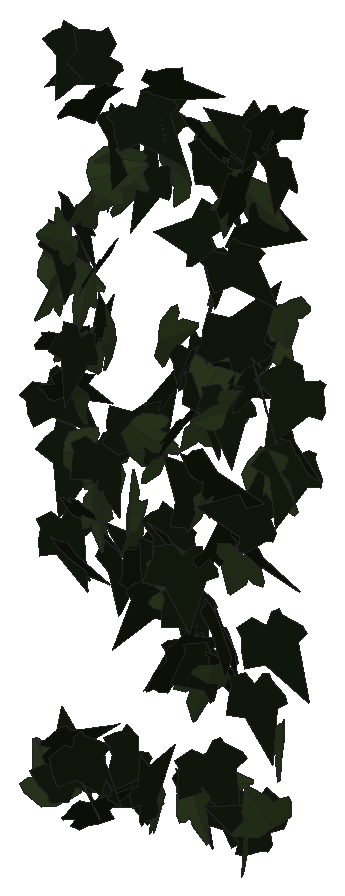
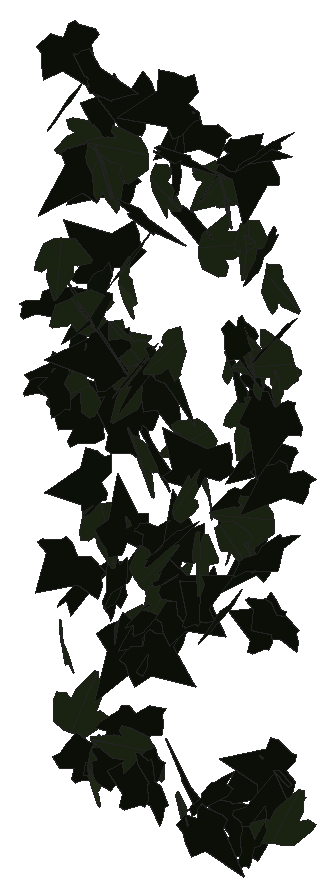
# SketchUp Ruby script. Lengths in inches.
U = 1.inch
M = Sketchup.active_model
def pt(a) = Geom::Point3d.new(a.map { |v| v * U })
def face(e, loops, mat)
  f = e.add_face(loops[0].map { |a| pt(a) })
  loops[1..].each { |l| e.add_face(l.map { |a| pt(a) }).erase! }
  f.material = f.back_material = mat if mat
  f
end
# faces: each face lists its corners as indices into pts; further lists are holes
def faces(e, pts, list, mat = nil) = list.each { |f| face(e, (f[0].is_a?(Array) ? f : [f]).map { |l| l.map { |i| pts[i] } }, mat) }
# xy, xz, yz: faces in a plane at the given z, y or x. An outline is a flat list of corners, or four numbers for a rectangle; further outlines are holes
def ring(l) = l.size == 4 ? [[l[0], l[1]], [l[2], l[1]], [l[2], l[3]], [l[0], l[3]]] : l.each_slice(2).to_a
def flat(e, list, mat, &to3) = list.each { |f| face(e, (f[0].is_a?(Array) ? f : [f]).map { |l| ring(l).map { |u, v| to3.(u, v) } }, mat) }
def xy(e, z, list, mat = nil) = flat(e, list, mat) { |x, y| [x, y, z] }
def xz(e, y, list, mat = nil) = flat(e, list, mat) { |x, z| [x, y, z] }
def yz(e, x, list, mat = nil) = flat(e, list, mat) { |y, z| [x, y, z] }
def lines(e, pts, list) = list.each { |a, b| e.add_line(pt(pts[a]), pt(pts[b])) }
# prism: a flat outline (further loops are holes) pulled along v
def prism(e, loops, v, mat = nil)
  f = face(e, loops, mat); d = Geom::Vector3d.new(v.map { |x| x * U })
  f.pushpull(f.normal.samedirection?(d) ? d.length : -d.length)
end
def box(e, o, s, mat = nil) = prism(e, [[o, [o[0] + s[0], o[1], o[2]], [o[0] + s[0], o[1] + s[1], o[2]], [o[0], o[1] + s[1], o[2]]]], [0, 0, s[2]], mat)
def at(x, y, z, deg = 0) = Geom::Transformation.translation(pt([x, y, z])) * Geom::Transformation.rotation(ORIGIN, Z_AXIS, deg.degrees)
def axes(o, x, y, z) = Geom::Transformation.new([*x, 0, *y, 0, *z, 0, *pt(o).to_a, 1])
def part(name) = M.definitions.add(name)
# library, detail: a bought-in or finely detailed component or shape, given as its bounding box
def library(name, o, s) = part(name).tap { |d| box(d.entities, o, s) }
def detail(e, o, s) = box(e.add_group.entities, o, s)
def put(e, d, t, mat = nil) = e.add_instance(d, t).tap { |i| i.material = mat if mat }
def group(e, t, mat = nil) = e.add_group.tap { |g| g.transformation = t; g.material = mat if mat }.entities
root = M.entities
M.materials.add("efeu1").color = [18, 25, 13]
M.materials.add("efeu2").color = [43, 57, 29]
c1 = part("ivyleaf_9")
p = [[1.54,2.16,1.25],[1.36,2.04,1.19],[-0.21,0.99,0.68],[-0.71,1.11,0.82],[-0.85,0.86,0.67],[-0.8,0.17,0.21],
  [-0.9,-0.01,0.1],[-0.67,-0.16,-0.02],[-0.08,-0.08,-0.05],[-0.03,-0.6,-0.4],[0.65,-0.88,-0.66],[0.83,-0.6,-0.49],
  [1.29,-0.42,-0.43],[1.8125,-0.07,-0.26],[1.21,0.44,0.15]]
faces(c1.entities,p,[[0,1,2,3,4,5,6,7,8,9,10,11,12,13,14]],"efeu1")
c2 = part("ivyleaf_10")
p = [[0,0.5,-0.03],[-0.0625,2.02,-0.43],[-0.19,2.01,-0.46],[-0.54,1.05,-0.29],[-0.52,0.625,-0.18],[-0.83,0.76,-0.28],
  [-1.16,0.64,-0.33],[-1.15,0.33,-0.24],[-0.77,-0.39,0.02],[-0.3,-0.51,0.16],[0.04,-0.48,0.23],[-0.02,2.01,-0.4375],
  [-0.06,2.01,-0.43],[0.04,-0.49,0.23],[0.67,-0.49,0.14],[1.38,0.36,-0.2],[1.375,0.51,-0.24],[0.81,0.65,-0.19],
  [0.62,0.59,-0.15],[0.6,1.09,-0.28],[0.5,1.23,-0.31]]
faces(c2.entities,p,[[0,1,2,3,4,5,6,7,8,9,10],[11,12,0,13,14,15,16,17,18,19,20]],"efeu2")
put(root,c1,axes([566.55,125.93,235.69],[0.48695,-0.82806,0.32776],[0.14634,-0.29408,-0.96038],[0.87846,0.508,-0.0217]))
put(root,c1,axes([576.53,125.82,215.84],[0.2139,-1.10488,-0.24681],[-0.04324,0.24302,-1.12539],[1.13129,0.2182,0.00365]))
put(root,c2,axes([566.59,125.89,226.53],[-0.60718,0.06455,0.81247],[0.77355,-0.27349,0.59981],[0.25672,0.97672,0.11426]))
put(root,c2,axes([570.2,125.27,222.05],[0.76688,-0.41695,0.66634],[-0.54996,0.38051,0.87104],[-0.56161,-0.94198,0.05691]))
put(root,c2,axes([569.02,125.73,238.55],[0.64031,-0.81411,-0.13122],[-0.06589,0.11509,-1.03557],[0.82198,0.6434,0.01921]))
put(root,c2,axes([566.38,125.54,234.33],[-0.24169,0.05211,0.98861],[-0.9899,0.00032,-0.24202],[-0.01269,-1.01773,0.05054]))
put(root,c1,axes([575.42,125.39,236.79],[-0.1494,-0.23257,-1.00547],[0.54358,0.84586,-0.27642],[0.87725,-0.56374,0.00004]))
put(root,c2,axes([568.43,125.38,238.32],[0.39007,-0.07838,-0.94898],[0.92972,0.25294,0.36126],[0.20575,-0.99435,0.1667]))
put(root,c2,axes([568.24,126.27,229.74],[-0.30866,0.37768,0.92115],[0.60809,-0.69208,0.48752],[0.78828,0.68177,-0.0154]))
put(root,c1,axes([573.6,126.06,224.64],[0.40899,-0.33145,1.27453],[1.0095,-0.77814,-0.52631],[0.84571,1.08914,0.01185]))
put(root,c1,axes([576.58,126.56,223.89],[-0.20394,-0.14405,1.19482],[-0.97775,-0.68673,-0.24968],[0.70168,-0.99879,-0.00065]))
put(root,c1,axes([566.02,125.15,209.54],[0.25416,0.7736,-0.6093],[0.12603,0.59854,0.81251],[0.97664,-0.27856,0.05372]))
put(root,c1,axes([566.63,126.13,229.29],[-0.79593,-0.23059,-0.56353],[0.55679,0.09972,-0.82721],[0.24642,-0.97012,0.04892]))
put(root,c1,axes([566.72,125.64,209.44],[-0.18209,-0.27365,-1.02257],[0.61599,0.81643,-0.32817],[0.86087,-0.64207,0.01853]))
put(root,c2,axes([567.29,126.3,221.61],[0.71805,-0.30645,0.80688],[0.75671,-0.28134,-0.78025],[0.41516,1.04283,0.02661]))
put(root,c2,axes([574.77,126.66,228.54],[0.04325,0.06862,-1.05561],[-0.6146,-0.85825,-0.08097],[-0.86097,0.61611,0.00477]))
put(root,c2,axes([567.42,125.78,236.6],[-0.02899,-0.93369,-0.40921],[0.04456,0.40782,-0.93368],[1.01845,-0.04442,0.0292]))
put(root,c1,axes([575.56,125.26,239.25],[0.0199,-0.13283,1.13701],[0.46635,1.03948,0.11327],[-1.04545,0.46116,0.07217]))
put(root,c1,axes([567.06,125.57,206.29],[0.42568,0.88116,-0.3023],[0.13152,0.27219,0.97859],[0.92224,-0.44554,-0.00002]))
put(root,c1,axes([575.42,125.49,232.03],[-0.39089,-0.25075,1.19291],[1.07257,0.52453,0.46171],[-0.57923,1.14048,0.04993]))
put(root,c2,axes([565.49,126.1,206.94],[0.54037,1.0486,0.35028],[-0.1768,-0.3029,1.17951],[1.09133,-0.56828,0.01765]))
put(root,c2,axes([576.62,126.57,209.03],[-0.61666,-0.76684,-0.5738],[-0.36437,-0.44329,0.98402],[-0.88573,0.71625,-0.00531]))
put(root,c1,axes([572.86,127.04,215.16],[-0.33751,-0.47663,1.00169],[-0.09803,-1.03012,-0.52318],[1.10497,-0.23698,0.25955]))
put(root,c1,axes([572.33,126.0625,227.39],[-0.40754,0.83497,-0.34004],[0.1324,-0.31369,-0.92895],[-0.89178,-0.42815,0.01748]))
put(root,c2,axes([568.79,125.87,238.98],[-0.73084,-0.35841,-0.61342],[0.55355,0.26436,-0.81398],[0.44533,-0.9168,0.00509]))
put(root,c1,axes([568.41,127.04,239.49],[0.02553,-0.91032,0.80064],[0.06943,-0.79841,-0.90999],[1.21033,0.065,0.03531]))
put(root,c1,axes([572.02,126.47,220.29],[-0.37583,-0.89923,-0.48626],[0.23868,0.42658,-0.97333],[0.99403,-0.44241,0.04986]))
put(root,c1,axes([566.43,126.08,207.5],[-0.81879,-0.63423,0.4677],[0.36984,0.28629,1.03569],[-0.69585,0.89844,0.00014]))
put(root,c1,axes([574.4,126.52,228.99],[-0.60036,-0.48133,-0.70867],[0.63785,0.32653,-0.76214],[0.57187,-0.8695,0.10609]))
put(root,c2,axes([573.34,126.6,215.01],[-0.27552,-1.10426,0.25761],[-0.0469,-0.25378,-1.13801],[1.13294,-0.27905,0.01554]))
put(root,c1,axes([566.44,126.06,221.1],[1.0125,-0.01233,-0.06006],[-0.05991,0.01285,-1.0125],[0.01307,1.0142,0.0121]))
put(root,c2,axes([567.98,125.74,221.92],[-0.41154,0.56329,0.78885],[-0.44282,0.6531,-0.69737],[-0.86226,-0.60426,-0.01837]))
put(root,c2,axes([572.39,126.54,208.76],[0.75051,-0.12421,0.72321],[0.72656,-0.01921,-0.75729],[0.10285,1.04209,0.07224]))
put(root,c1,axes([573.55,127.12,217.18],[0.22616,-0.7876,0.74488],[0.22085,-0.71148,-0.81935],[1.06131,0.31588,0.01177]))
put(root,c1,axes([572.89,125.99,223.88],[-0.66822,0.17931,-0.96748],[-0.97464,0.03991,0.68057],[0.13507,1.17513,0.12451]))
put(root,c1,axes([573.9,127.12,216.33],[-0.02798,-0.17929,1.15073],[0.38083,-1.08919,-0.16044],[1.10058,0.37233,0.08478]))
put(root,c2,axes([564.68,127.11,230.85],[-0.12079,0.38531,-0.91012],[-0.08997,-0.91737,-0.37644],[-0.98422,0.03657,0.14611]))
put(root,c1,axes([572.1,125.44,215.76],[-0.21963,0.51256,-1.13394],[-0.48694,1.02425,0.5573],[1.14518,0.53383,0.01949]))
put(root,c1,axes([567.19,126.67,223.98],[0.16706,-0.9687,-0.45375],[-0.04865,0.4519,-0.98265],[1.0686,0.17201,0.0262]))
put(root,c1,axes([572.7,126.8,241.17],[0.54792,-0.47737,0.79131],[0.68274,-0.41089,-0.72063],[0.62282,0.87038,0.09381]))
put(root,c1,axes([576.93,126.91,243.52],[-0.03947,0.6301,-0.86428],[0.08915,-0.85992,-0.631],[-1.06586,-0.09526,-0.02077]))
put(root,c1,axes([569.62,126.46,241.48],[-0.05261,-0.49736,-0.98113],[0.53907,0.84456,-0.45703],[0.95885,-0.5021,0.20311]))
put(root,c2,axes([572.93,126.75,224.26],[1.03754,-0.62532,-0.1728],[-0.1373,0.10691,-1.21124],[0.63406,1.04639,0.02048]))
put(root,c2,axes([566.25,126.95,231.75],[1.07502,-0.563,0.17863],[0.16841,-0.06341,-1.21333],[0.56615,1.08792,0.02172]))
put(root,c1,axes([565.42,126.14,226.72],[0.79539,0.4763,0.35874],[0.31504,0.1721,-0.927],[-0.50627,0.85541,-0.01324]))
put(root,c2,axes([569.68,126.48,225.85],[-0.52176,-0.24041,-0.78625],[0.74838,0.24674,-0.57207],[0.34047,-0.91079,0.05256]))
put(root,c1,axes([575.82,126.51,241.78],[-0.35768,0.23247,1.0327],[-0.81807,0.63106,-0.4254],[-0.67177,-0.89228,-0.03181]))
put(root,c2,axes([576.09,126.71,226.08],[0.68938,0.09709,0.99761],[0.96687,0.25479,-0.69293],[-0.26425,1.18556,0.06722]))
put(root,c1,axes([565.89,127.39,206.74],[0.28335,-0.56852,0.83965],[0.35633,-0.76039,-0.6351],[0.94934,0.45509,-0.01223]))
put(root,c2,axes([576.76,127.2,213.05],[0.61421,-0.43975,0.62161],[0.52256,-0.33742,-0.75505],[0.55381,0.8061,0.02305]))
put(root,c1,axes([569.95,127.41,217.7],[-0.0935,0.32339,-1.06895],[0.29821,-1.02651,-0.33663],[-1.07624,-0.31252,-0.00041]))
put(root,c1,axes([572.625,127.24,228.53],[0.34899,-1.02825,0.09986],[0.01563,-0.10014,-1.08573],[1.03297,0.34891,-0.01731]))
put(root,c2,axes([573.16,126.42,227.4],[-0.44802,-0.72054,-0.65323],[0.34786,0.55291,-0.84846],[0.90823,-0.56721,0.00274]))
put(root,c1,axes([575.7,127.59,228.48],[-0.0528,-0.18333,1.15102],[0.27958,-1.12055,-0.16565],[1.1315,0.26833,0.09464]))
put(root,c1,axes([571.6875,126.7,229.11],[-0.73745,0.85299,0.01221],[-0.01628,0.00207,-1.12752],[-0.85292,-0.73755,0.01097]))
put(root,c1,axes([577.68,127.57,230.38],[-0.65017,-0.90154,0.15842],[-0.08946,-0.13081,-1.11152],[0.91097,-0.65628,0.00392]))
put(root,c1,axes([565.24,127.1,217.77],[0.47213,-0.42368,0.70592],[0.59946,-0.38089,-0.62953],[0.56434,0.75905,0.07813]))
put(root,c1,axes([575.04,126.9,221.74],[0.88268,-0.36713,0.45083],[0.42271,-0.15749,-0.95586],[0.39919,0.97856,0.01531]))
put(root,c1,axes([572.99,127.14,240.24],[0.63784,-1.0423,-0.19078],[-0.10369,0.16021,-1.22197],[1.05453,0.6462,-0.00477]))
put(root,c1,axes([569.46,126.87,207.31],[-0.4334,0.76744,0.77397],[0.38828,-0.66955,0.88133],[1.01844,0.58185,-0.00665]))
put(root,c2,axes([567.88,127.86,236.55],[-0.00058,-0.21122,1.13229],[-0.06324,-1.13057,-0.21093],[1.15008,-0.06228,-0.01103]))
put(root,c1,axes([577.27,127.5625,226.59],[-0.43705,-0.97645,-0.02745],[0.01193,0.02474,-1.0698],[0.97676,-0.43721,0.00078]))
put(root,c1,axes([569.82,127.57,220.05],[1.08973,-0.28345,-0.41835],[0.40627,-0.09994,1.12597],[-0.3005,-1.16298,0.0052]))
put(root,c2,axes([575.33,127.05,239.0625],[-0.59983,0.10924,-0.86829],[0.85577,-0.14699,-0.60967],[-0.18307,-1.04504,-0.00501]))
put(root,c1,axes([566.54,126.59,240.9],[0.26965,0.98217,-0.04078],[-0.01633,-0.03781,-1.0185],[-0.98288,0.27008,0.00573]))
put(root,c1,axes([572.92,127.07,236.15],[-0.69091,0.40119,0.58922],[-0.57644,0.16828,-0.79051],[-0.41935,-0.89232,0.11584]))
put(root,c1,axes([572.99,126.93,210.64],[-0.03243,-0.78656,-0.84268],[0.02364,0.84238,-0.78719],[1.15249,-0.03941,-0.00757]))
put(root,c1,axes([564.71,127.7,232.78],[0.06963,-0.96869,0.27036],[0.04177,-0.26799,-0.97094],[1.00484,0.07826,0.02162]))
put(root,c1,axes([576.2,127.82,240.77],[0.12115,-0.89375,0.53404],[0.07342,-0.52897,-0.90193],[1.03856,0.14165,0.00146]))
put(root,c1,axes([565.33,126.7,228.8],[0.63514,0.83868,-0.24486],[-0.16379,-0.18307,-1.05185],[-0.8582,0.65562,0.01953]))
put(root,c2,axes([565.97,127.02,230.13],[0.68303,-0.65518,0.33657],[-0.25092,0.22459,0.9464],[-0.69252,-0.72758,-0.01094]))
put(root,c1,axes([570.49,128.01,220.54],[-0.26353,-0.92701,0.44825],[-0.07262,-0.44481,-0.9626],[1.02713,-0.26929,0.04695]))
put(root,c2,axes([565.83,126.99,223.17],[-0.05377,-0.07689,-1.07137],[1.0559,0.193,-0.06684],[0.19705,-1.05522,0.06584]))
put(root,c2,axes([572.98,126.95,228.9375],[0.87522,0.18903,-0.49509],[0.45765,0.21239,0.89012],[0.26722,-0.98286,0.09713]))
put(root,c1,axes([564.36,126.95,225.89],[0.02578,-0.44563,-0.93884],[0.24069,0.91615,-0.42826],[1.01098,-0.20675,0.1259]))
put(root,c1,axes([567.33,126.5625,229.5625],[-0.07228,0.46618,0.92228],[-0.22421,0.89543,-0.47018],[-1.00879,-0.23242,0.03842]))
put(root,c2,axes([574.53,127.96,207.79],[0.47362,-0.64672,0.95066],[0.667,-0.68294,-0.79689],[0.93654,0.81343,0.08678]))
put(root,c1,axes([565.16,128.0625,242.35],[-0.33346,-0.89236,0.41066],[0.04507,-0.44712,-0.93499],[0.98128,-0.28271,0.1825]))
put(root,c1,axes([575.55,127.82,207.61],[-0.11922,0.01372,1.05028],[-0.98065,-0.38015,-0.10635],[0.37631,-0.9863,0.05559]))
put(root,c1,axes([574.34,127.7,208.23],[-0.24472,-0.24105,-0.9004],[-0.53737,-0.72416,0.33992],[-0.76161,0.5884,0.04948]))
put(root,c1,axes([569.67,127.89,240.3],[0.2498,-0.14624,-1.14518],[1.11616,-0.2688,0.2778],[-0.295,-1.14087,0.08134]))
put(root,c1,axes([567.43,128.03,217.83],[0.0807,-0.88599,0.51674],[0.13376,-0.50481,-0.88645],[1.01691,0.13671,0.07559]))
put(root,c1,axes([568.14,128.1,208.74],[-0.28832,-0.7516,0.52577],[-0.20018,-0.48629,-0.80494],[0.89514,-0.35084,-0.01066]))
put(root,c2,axes([570.04,127.35,207.32],[0.5771,-0.74826,-0.2803],[-0.16599,0.22596,-0.94494],[0.78161,0.60046,0.00629]))
put(root,c2,axes([566.09,127.18,228.65],[-0.60754,-0.84557,-0.34477],[0.1746,0.2989,-1.04074],[0.89631,-0.63137,-0.03096]))
put(root,c1,axes([575.96,127.39,217.84],[-0.32485,-0.39276,-1.11955],[0.85668,0.7254,-0.50306],[0.82082,-0.91253,0.08196]))
put(root,c1,axes([570.15,126.9,242.66],[0.74265,0.21526,0.69483],[0.66982,0.18485,-0.77319],[-0.28366,1.00007,-0.00665]))
put(root,c1,axes([564.54,127.5625,218.97],[-0.35539,-0.36584,-0.94495],[0.84571,0.4445,-0.49016],[0.55816,-0.90645,0.14102]))
put(root,c1,axes([575.66,127,230.43],[-0.81261,0.88012,0.56704],[-0.3647,0.43489,-1.19764],[-0.9814,-0.89036,-0.02446]))
put(root,c2,axes([569.03,127.14,220.78],[0.14913,-0.9081,-0.59435],[-0.13956,0.57891,-0.91952],[1.0763,0.20089,-0.03688]))
put(root,c2,axes([573.96,127.77,238.4],[0.0177,-1.05257,0.22896],[0.03693,-0.22827,-1.05223],[1.07656,0.02514,0.03233]))
put(root,c1,axes([571.56,127.91,214.99],[-0.04478,0.28385,-0.9545],[-0.1877,-0.94074,-0.27095],[-0.97796,0.16756,0.09571]))
put(root,c1,axes([566.71,127.48,232.61],[-0.51233,0.78708,-0.34025],[0.20556,-0.27206,-0.93886],[-0.83247,-0.55157,-0.02243]))
put(root,c1,axes([571.71,127.8125,208.08],[0.51056,-0.44577,0.91835],[0.75279,-0.52911,-0.67535],[0.68948,0.90779,0.05732]))
put(root,c2,axes([572.41,127.3125,209.3],[0.07664,-0.07733,-1.08822],[1.0796,0.16241,0.06449],[0.15704,-1.07876,0.08772]))
put(root,c2,axes([570.71,127.88,217.6],[0.12689,0.91034,0.6083],[-0.1072,-0.5991,0.91893],[1.08961,-0.16496,0.01957]))
put(root,c1,axes([574.35,127.41,231.82],[1.03325,-0.47011,-0.23639],[-0.21978,0.08772,-1.13512],[0.47809,1.05631,-0.01094]))
put(root,c2,axes([574.32,127.57,220.54],[-0.98817,-0.16084,0.47575],[-0.46977,-0.07516,-1.00117],[0.17753,-1.09415,-0.00116]))
put(root,c1,axes([568.86,127.21,224.46],[-0.57981,-0.08986,0.99776],[0.98198,0.17722,0.5866],[-0.1983,1.14031,-0.01254]))
put(root,c1,axes([572.83,127.71,220.04],[0.41953,0.74012,0.55673],[-0.39664,-0.40871,0.84224],[0.8369,-0.56472,0.12008]))
put(root,c1,axes([569.42,127.92,237.86],[-0.91942,-0.0918,-0.41817],[0.41368,0.06471,-0.92375],[0.11029,-1.00798,-0.02122]))
put(root,c1,axes([575.49,126.83,237.86],[0.05885,-0.00993,-1.16856],[-0.33893,1.1196,-0.02658],[1.11837,0.33983,0.05343]))
put(root,c1,axes([566.35,128.32,242.09],[-0.63325,-0.47169,0.62719],[-0.52232,-0.34815,-0.7892],[0.5857,-0.82046,-0.02569]))
put(root,c2,axes([564.27,127.35,231.75],[0.29929,0.1229,1.15898],[1.021,0.54939,-0.32192],[-0.56204,1.06347,0.03237]))
put(root,c2,axes([571.38,128.01,218.78],[-0.72244,-0.18182,-0.67944],[-0.64774,-0.20757,0.74428],[-0.27409,0.96978,0.03192]))
put(root,c2,axes([571.29,127.34,238.39],[0.07642,-0.09058,-1.08147],[-0.84814,0.6714,-0.11617],[0.67708,0.85125,-0.02346]))
put(root,c1,axes([571.06,128.02,208.49],[-0.19401,-0.09533,-1.1181],[1.10653,0.1725,-0.20671],[0.18667,-1.12162,0.06324]))
put(root,c1,axes([564.74,128.46,222.4375],[-0.29496,-1.09975,0.1703],[-0.03975,-0.16566,-1.13861],[1.11215,-0.2976,0.00447]))
put(root,c1,axes([569.67,127.91,218.1],[0.0934,-0.00701,1.13133],[-1.08032,0.33653,0.09128],[-0.33595,-1.08415,0.02102]))
put(root,c2,axes([572.33,128.43,233.25],[0.49785,-0.5565,0.79807],[0.49664,-0.62553,-0.746],[0.83663,0.70247,-0.03206]))
put(root,c1,axes([571.02,127.98,217.39],[0.20928,-0.9545,-0.35769],[-0.03834,0.35752,-0.97649],[1.0186,0.20957,0.03674]))
put(root,c2,axes([566.96,127.84,222.44],[0.74641,-0.17644,-0.64816],[-0.61816,0.19882,-0.76598],[0.26292,0.96836,0.03917]))
put(root,c2,axes([568.97,128.58,223.53],[-0.27126,0.49807,1.00316],[0.34702,-0.94399,0.56253],[1.06488,0.43449,0.07222]))
put(root,c1,axes([568.79,127.35,217.88],[-0.1384,-0.30348,0.95173],[0.48402,0.82013,0.33191],[-0.87386,0.50233,0.0331]))
put(root,c2,axes([570.5,127.13,230.37],[-0.04191,-0.2334,-1.06216],[0.25067,1.03225,-0.23672],[1.05822,-0.25376,0.01401]))
put(root,c1,axes([570.125,128.29,240.77],[-0.9294,0.07374,0.34309],[-0.35092,-0.19852,-0.90795],[0.00116,-0.97061,0.21177]))
put(root,c1,axes([572.14,128.56,234.53],[0.15494,-0.91076,0.43693],[0.08325,-0.42902,-0.9238],[1.0067,0.17565,0.00915]))
put(root,c1,axes([576.18,128.06,226.89],[0.27814,0.01888,-0.94334],[0.91876,0.21843,0.27527],[0.21476,-0.95893,0.04413]))
put(root,c1,axes([568.45,128.03,207.375],[0.10891,0.10245,-1.06024],[-0.86523,-0.6131,-0.14812],[-0.62127,0.87182,0.02042]))
put(root,c2,axes([576.44,127.89,233.42],[-0.53411,-0.91102,-0.14357],[0.07609,0.12182,-1.05604],[0.91912,-0.53949,0.00399]))
put(root,c2,axes([573.85,128.25,239.28],[0.71627,-0.79352,0.09931],[0.06442,-0.07563,-1.06898],[0.79711,0.71916,-0.00284]))
put(root,c1,axes([571.27,127.89,229.57],[0.4964,-0.78547,-0.56603],[-0.25265,0.50896,-0.92784],[0.93462,0.55476,0.04981]))
put(root,c1,axes([572.5,127.66,214.98],[1.07407,0.16301,-0.25278],[-0.24959,-0.04004,-1.08637],[-0.16784,1.10269,-0.00208]))
put(root,c2,axes([572.13,128.02,239.98],[-0.10379,-0.0993,-1.15253],[1.15362,-0.0946,-0.09574],[-0.08569,-1.15332,0.10708]))
put(root,c1,axes([573.4,127.76,229.06],[0.81645,0.00088,0.77181],[0.77127,-0.04313,-0.81582],[0.02899,1.12269,-0.03195]))
put(root,c2,axes([575.06,128.35,231.34],[0.84206,0.61318,-0.5629],[-0.47623,-0.3018,-1.04117],[-0.68268,0.96687,0.03199]))
